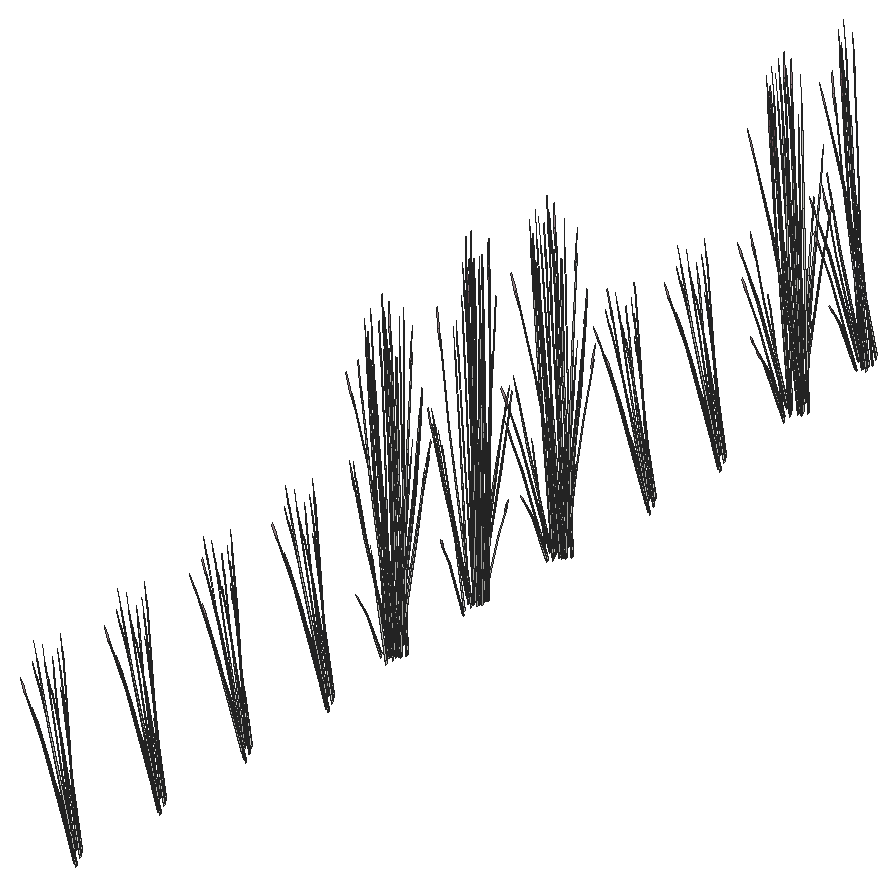
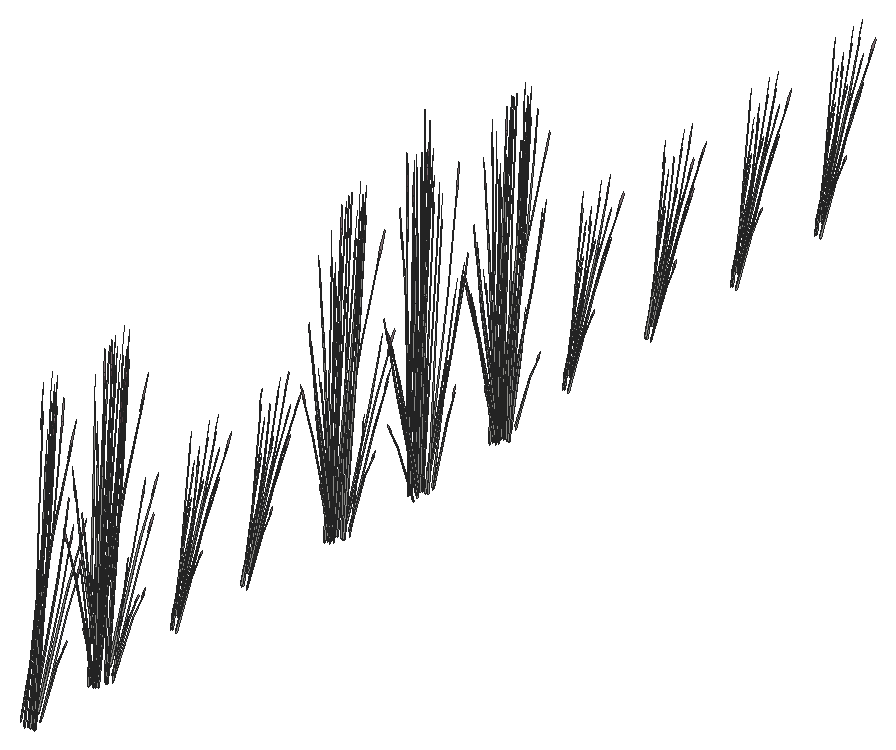
# SketchUp Ruby script. Lengths in inches.
U = 1.inch
M = Sketchup.active_model
def pt(a) = Geom::Point3d.new(a.map { |v| v * U })
def face(e, loops, mat)
  f = e.add_face(loops[0].map { |a| pt(a) })
  loops[1..].each { |l| e.add_face(l.map { |a| pt(a) }).erase! }
  f.material = f.back_material = mat if mat
  f
end
# faces: each face lists its corners as indices into pts; further lists are holes
def faces(e, pts, list, mat = nil) = list.each { |f| face(e, (f[0].is_a?(Array) ? f : [f]).map { |l| l.map { |i| pts[i] } }, mat) }
# xy, xz, yz: faces in a plane at the given z, y or x. An outline is a flat list of corners, or four numbers for a rectangle; further outlines are holes
def ring(l) = l.size == 4 ? [[l[0], l[1]], [l[2], l[1]], [l[2], l[3]], [l[0], l[3]]] : l.each_slice(2).to_a
def flat(e, list, mat, &to3) = list.each { |f| face(e, (f[0].is_a?(Array) ? f : [f]).map { |l| ring(l).map { |u, v| to3.(u, v) } }, mat) }
def xy(e, z, list, mat = nil) = flat(e, list, mat) { |x, y| [x, y, z] }
def xz(e, y, list, mat = nil) = flat(e, list, mat) { |x, z| [x, y, z] }
def yz(e, x, list, mat = nil) = flat(e, list, mat) { |y, z| [x, y, z] }
def lines(e, pts, list) = list.each { |a, b| e.add_line(pt(pts[a]), pt(pts[b])) }
# prism: a flat outline (further loops are holes) pulled along v
def prism(e, loops, v, mat = nil)
  f = face(e, loops, mat); d = Geom::Vector3d.new(v.map { |x| x * U })
  f.pushpull(f.normal.samedirection?(d) ? d.length : -d.length)
end
def box(e, o, s, mat = nil) = prism(e, [[o, [o[0] + s[0], o[1], o[2]], [o[0] + s[0], o[1] + s[1], o[2]], [o[0], o[1] + s[1], o[2]]]], [0, 0, s[2]], mat)
def at(x, y, z, deg = 0) = Geom::Transformation.translation(pt([x, y, z])) * Geom::Transformation.rotation(ORIGIN, Z_AXIS, deg.degrees)
def axes(o, x, y, z) = Geom::Transformation.new([*x, 0, *y, 0, *z, 0, *pt(o).to_a, 1])
def part(name) = M.definitions.add(name)
# library, detail: a bought-in or finely detailed component or shape, given as its bounding box
def library(name, o, s) = part(name).tap { |d| box(d.entities, o, s) }
def detail(e, o, s) = box(e.add_group.entities, o, s)
def put(e, d, t, mat = nil) = e.add_instance(d, t).tap { |i| i.material = mat if mat }
def group(e, t, mat = nil) = e.add_group.tap { |g| g.transformation = t; g.material = mat if mat }.entities
root = M.entities
M.materials.add("LightPink_Translucent").color = [144, 107, 117]
M.materials["LightPink_Translucent"].alpha = 0.75
c1 = part("blade")
p = [[2.15,0.21,22],[0,0.17,0],[0.09,0.45,0],[2.18,0.31,22],[2.29,0.31,22],[0.38,0.45,0],
  [2.48,0.24,33],[2.49,0.24,33],[2.48,0.22,33]]
faces(c1.entities,p,[[0,1,2,3],[4,5,2,3],[6,3,4,7],[8,0,3,6]])
c2 = part("seeds")
p = [[0.3,-0.1,1.38],[-0.01,-0.03,1.59],[-0.01,-0.03,0.03],[0.14,-0.07,-0.07],[0.29,-0.03,3],[0.15,0.01,3.11]]
faces(c2.entities,p,[[0,1,2,3],[1,0,4,5]],"LightPink_Translucent")
c3 = part("blade with seeds")
put(c3.entities,c1,at(0,0,0))
put(c3.entities,c2,axes([2.4,0.25,30.99],[1.5799,-0.05474,1.17369],[-0.12525,1.92788,0.29478],[-0.07173,-0.02425,1.56792]))
put(root,c3,axes([397.34,179.68,2.375],[-0.44133,0,0],[0,-0.52122,-0.51607],[0,-0.11871,1.63711]))
put(root,c3,axes([397.96,181,2.03],[-0.08291,-0.40636,-0.30978],[0.32928,-0.11539,0.30978],[-0.06638,-0.04686,1.38974]))
put(root,c3,axes([398.54,276.34,2.02],[-0.33032,-0.23318,-0.49651],[0.19744,-0.41812,0],[-0.07523,-0.05311,1.57504]))
put(root,c3,axes([398.4,272.86,1.49],[-0.03419,0.06144,1.76342],[-0.3455,0.13246,-0.26939],[-0.08346,-0.12049,0.30037]))
put(root,c3,axes([397.78,181.42,4.53],[-0.23881,0.24554,-0.35414],[-0.22606,-0.28036,0.4572],[-0.0344,0.14245,0.87481]))
put(root,c3,axes([398.2,290.38,2.59],[-0.02137,0.15256,1.43002],[-0.31245,0.12771,-0.30754],[-0.07303,-0.19719,0.61141]))
put(root,c3,axes([398.3,290.78,3.875],[0.08068,0.14973,1.71376],[-0.3728,0.12606,0.13857],[-0.08426,-0.23506,0.73262]))
put(root,c3,axes([398.74,276.62,2.375],[-0.22066,0.46731,0],[-0.36918,-0.26061,-0.51607],[-0.08408,-0.05936,1.63711]))
put(root,c3,axes([396.73,201.81,2.82],[0.32063,-0.08258,0.06507],[0.07371,0.33271,-0.86304],[-0.02033,0.16842,0.7736]))
put(root,c3,axes([398.24,200.32,2.67],[0.04113,0.53214,-0.29095],[-0.42835,0.03218,-0.50002],[-0.07543,0.07088,1.59708]))
put(root,c3,axes([397.28,199.42,2.1],[-0.14494,-0.47823,-0.69835],[0.41752,-0.17223,-0.18329],[-0.01602,-0.16194,1.54149]))
put(root,c3,axes([398.13,221,2.59],[0.11138,-0.07357,1.43002],[0.27499,0.22183,-0.30754],[-0.08185,0.19194,0.61141]))
put(root,c3,axes([400.46,100.5625,3.875],[0.14639,-0.01056,1.71376],[-0.09712,0.45778,0.13857],[-0.20862,-0.02831,0.73262]))
put(root,c3,axes([400.46,120.65,3.875],[0.14639,-0.01056,1.71376],[-0.09712,0.45778,0.13857],[-0.20862,-0.02831,0.73262]))
put(root,c3,axes([400.46,141.1,3.875],[0.14639,-0.01056,1.71376],[-0.09712,0.45778,0.13857],[-0.20862,-0.02831,0.73262]))
put(root,c3,axes([400.46,160.8,3.875],[0.14639,-0.01056,1.71376],[-0.09712,0.45778,0.13857],[-0.20862,-0.02831,0.73262]))
put(root,c3,axes([400.46,237.64,3.875],[0.14639,-0.01056,1.71376],[-0.09712,0.45778,0.13857],[-0.20862,-0.02831,0.73262]))
put(root,c3,axes([400.46,254.51,3.875],[0.14639,-0.01056,1.71376],[-0.09712,0.45778,0.13857],[-0.20862,-0.02831,0.73262]))
put(root,c3,axes([399,180.6875,2.06],[-0.23773,0.35053,-0.62353],[-0.29532,-0.31785,-0.16365],[-0.09526,0.08744,1.37633]))
put(root,c3,axes([397.93,197.92,4.68],[-0.34695,-0.11691,-0.51099],[0.11892,-0.40083,-0.3958],[-0.03181,-0.16138,0.97773]))
put(root,c3,axes([397.97,216.8,2.13],[-0.10181,0.3808,-0.03893],[-0.31336,-0.11714,-0.17649],[-0.04758,-0.06228,0.58215]))
put(root,c3,axes([398.44,290.7,4.53],[-0.05451,-0.37564,-0.35414],[0.31161,-0.09919,0.4572],[-0.0837,-0.10765,0.87481]))
put(root,c3,axes([397.57,292.6,2.375],[-0.44133,0,0],[0,-0.52122,-0.51607],[0,-0.11871,1.63711]))
put(root,c3,axes([397.68,179.54,2.33],[-0.32829,0.39208,0.30756],[-0.32849,-0.38796,-0.36492],[-0.01146,-0.11134,1.64885]))
put(root,c3,axes([397.29,200.9,3.875],[-0.00864,-0.17899,1.71376],[0.37441,0.11874,0.13857],[-0.02316,0.25508,0.73262]))
put(root,c3,axes([399.03,180.62,3.33],[0.305,0.18805,1.51261],[-0.29879,0.40513,0.59816],[-0.13384,-0.24012,1.26806]))
put(root,c3,axes([396.59,199.37,2.03],[0.24637,-0.29097,-0.30978],[0.24637,0.29097,0.30978],[0,-0.09372,1.38974]))
put(root,c3,axes([397.7,197.49,2.13],[-0.2439,0.26754,-0.03893],[-0.22348,-0.29302,-0.17649],[-0.01573,-0.08303,0.58215]))
put(root,c3,axes([398.4375,216.32,2.59],[-0.02137,0.15256,1.43002],[-0.31245,0.12771,-0.30754],[-0.07303,-0.19719,0.61141]))
put(root,c3,axes([397.87,177.21,2.77],[0.18411,0.16231,1.1486],[-0.26813,0.09757,0.84392],[-0.05737,-0.12474,0.25299]))
put(root,c3,axes([399.16,180.49,2.46],[-0.34464,-0.37536,-0.25192],[0.29,-0.42149,0.5513],[-0.0928,0.04391,1.68216]))
put(root,c3,axes([397.6,200.125,2.36],[0.44609,0.09826,0.45755],[-0.09078,0.55493,0.17955],[-0.06519,-0.05359,1.58856]))
put(root,c3,axes([398.54,216.72,3.875],[0.08068,0.14973,1.71376],[-0.3728,0.12606,0.13857],[-0.08426,-0.23506,0.73262]))
put(root,c3,axes([398.54,180.13,2.21],[-0.21202,-0.39143,-0.44739],[0.32115,-0.27564,0.21531],[-0.06861,-0.04843,1.43643]))
put(root,c3,axes([399.23,219.22,2.67],[-0.35635,0.30962,-0.29095],[-0.23697,-0.43749,-0.50002],[-0.08792,-0.04443,1.59708]))
put(root,c3,axes([398.34,277.29,2.59],[0.11138,-0.07357,1.43002],[0.27499,0.22183,-0.30754],[-0.08185,0.19194,0.61141]))
put(root,c3,axes([397.9375,181.16,5.34],[-0.00918,0.43138,-0.7886],[-0.38672,-0.02897,0.09517],[-0.04081,0.18275,1.11556]))
put(root,c3,axes([398.18,273.1,2.13],[-0.10181,0.3808,-0.03893],[-0.31336,-0.11714,-0.17649],[-0.04758,-0.06228,0.58215]))
put(root,c3,axes([398.67,216.64,4.53],[-0.05451,-0.37564,-0.35414],[0.31161,-0.09919,0.4572],[-0.0837,-0.10765,0.87481]))
put(root,c3,axes([397.93,182.38,2.77],[-0.00913,-0.2773,1.1486],[0.22824,0.19778,0.84392],[-0.04489,0.13217,0.25299]))
put(root,c3,axes([397.91,292.46,2.33],[-0.32829,0.39208,0.30756],[-0.32849,-0.38796,-0.36492],[-0.01146,-0.11134,1.64885]))
put(root,c3,axes([397.8,218.54,2.375],[-0.44133,0,0],[0,-0.52122,-0.51607],[0,-0.11871,1.63711]))
put(root,c3,axes([397.49,200.03,2.72],[-0.17124,0.42022,0.44739],[-0.35581,-0.20224,-0.21531],[0,-0.09687,1.43643]))
put(root,c3,axes([398.42,219.87,2.03],[-0.08291,-0.40636,-0.30978],[0.32928,-0.11539,0.30978],[-0.06638,-0.04686,1.38974]))
put(root,c3,axes([398.05,198,4.98],[-0.16845,-0.3792,-0.71045],[0.34676,-0.21133,0.08574],[-0.03939,-0.18322,1.00501]))
put(root,c3,axes([398.99,180.41,2.21],[-0.38326,0.02879,-0.44739],[-0.03466,-0.47788,0.21531],[-0.06861,0.04843,1.43643]))
put(root,c3,axes([399.26,293.55,3.33],[0.305,0.18805,1.51261],[-0.29879,0.40513,0.59816],[-0.13384,-0.24012,1.26806]))
put(root,c3,axes([398.24,220.29,4.53],[-0.23881,0.24554,-0.35414],[-0.22606,-0.28036,0.4572],[-0.0344,0.14245,0.87481]))
put(root,c3,axes([398.65,272.62,2.59],[-0.02137,0.15256,1.43002],[-0.31245,0.12771,-0.30754],[-0.07303,-0.19719,0.61141]))
put(root,c3,axes([400.52,101.37,3.875],[0.12246,-0.09864,1.71376],[0.1031,0.45582,0.13857],[-0.19225,0.10302,0.73262]))
put(root,c3,axes([400.52,121.46,3.875],[0.12246,-0.09864,1.71376],[0.1031,0.45582,0.13857],[-0.19225,0.10302,0.73262]))
put(root,c3,axes([400.52,141.91,3.875],[0.12246,-0.09864,1.71376],[0.1031,0.45582,0.13857],[-0.19225,0.10302,0.73262]))
put(root,c3,axes([400.52,161.6,3.875],[0.12246,-0.09864,1.71376],[0.1031,0.45582,0.13857],[-0.19225,0.10302,0.73262]))
put(root,c3,axes([400.52,238.44,3.875],[0.12246,-0.09864,1.71376],[0.1031,0.45582,0.13857],[-0.19225,0.10302,0.73262]))
put(root,c3,axes([400.52,255.32,3.875],[0.12246,-0.09864,1.71376],[0.1031,0.45582,0.13857],[-0.19225,0.10302,0.73262]))
put(root,c3,axes([398.75,273.01,3.875],[0.08068,0.14973,1.71376],[-0.3728,0.12606,0.13857],[-0.08426,-0.23506,0.73262]))
put(root,c3,axes([398.1,290.14,2.77],[0.18411,0.16231,1.1486],[-0.26813,0.09757,0.84392],[-0.05737,-0.12474,0.25299]))
put(root,c3,axes([399.4375,275.51,2.67],[-0.35635,0.30962,-0.29095],[-0.23697,-0.43749,-0.50002],[-0.08792,-0.04443,1.59708]))
put(root,c3,axes([400.14,102.14,2.59],[0.12266,0.03828,1.43002],[0.07906,0.39104,-0.30754],[-0.16661,0.0732,0.61141]))
put(root,c3,axes([400.14,122.24,2.59],[0.12266,0.03828,1.43002],[0.07906,0.39104,-0.30754],[-0.16661,0.0732,0.61141]))
put(root,c3,axes([400.14,142.68,2.59],[0.12266,0.03828,1.43002],[0.07906,0.39104,-0.30754],[-0.16661,0.0732,0.61141]))
put(root,c3,axes([400.14,162.38,2.59],[0.12266,0.03828,1.43002],[0.07906,0.39104,-0.30754],[-0.16661,0.0732,0.61141]))
put(root,c3,axes([400.14,239.22,2.59],[0.12266,0.03828,1.43002],[0.07906,0.39104,-0.30754],[-0.16661,0.0732,0.61141]))
put(root,c3,axes([400.14,256.1,2.59],[0.12266,0.03828,1.43002],[0.07906,0.39104,-0.30754],[-0.16661,0.0732,0.61141]))
put(root,c3,axes([397.37,201.01,2.47],[0.37926,-0.12378,0.17642],[0.09365,0.46065,0.35086],[-0.03382,-0.06712,1.60407]))
put(root,c3,axes([398.26,181.21,2.48],[0.33032,0.23318,0.49651],[-0.19744,0.41812,0],[-0.07523,-0.05311,1.57504]))
put(root,c3,axes([399.47,219.55,2.06],[-0.23773,0.35053,-0.62353],[-0.29532,-0.31785,-0.16365],[-0.09526,0.08744,1.37633]))
put(root,c3,axes([397.81,181.77,3.36],[0.00775,-0.24075,1.54345],[0.34877,0.12716,0.21329],[-0.03022,0.25658,0.72882]))
put(root,c3,axes([398.88,272.94,4.53],[-0.05451,-0.37564,-0.35414],[0.31161,-0.09919,0.4572],[-0.0837,-0.10765,0.87481]))
put(root,c3,axes([397.85,201.09,2.2],[-0.35581,-0.20937,0],[0.17124,-0.43505,0],[0,0,1.62707]))
put(root,c3,axes([398.01,274.84,2.375],[-0.44133,0,0],[0,-0.52122,-0.51607],[0,-0.11871,1.63711]))
put(root,c3,axes([398.63,276.16,2.03],[-0.08291,-0.40636,-0.30978],[0.32928,-0.11539,0.30978],[-0.06638,-0.04686,1.38974]))
put(root,c3,axes([398.57,180.36,2.4375],[0.09355,-0.55261,-0.23429],[0.44354,0.09633,0.51271],[-0.0775,-0.07631,1.5644]))
put(root,c3,axes([398.14,218.4,2.33],[-0.32829,0.39208,0.30756],[-0.32849,-0.38796,-0.36492],[-0.01146,-0.11134,1.64885]))
put(root,c3,axes([398.68,201.61,2.375],[0.22066,0.46731,0],[-0.36918,0.26061,-0.51607],[-0.08408,0.05936,1.63711]))
put(root,c3,axes([401.22,100.89,3.34],[0.10032,-0.06746,1.77064],[0.0346,0.47103,0.13857],[-0.2173,0.0625,0.63284]))
put(root,c3,axes([401.22,120.98,3.34],[0.10032,-0.06746,1.77064],[0.0346,0.47103,0.13857],[-0.2173,0.0625,0.63284]))
put(root,c3,axes([401.22,141.43,3.34],[0.10032,-0.06746,1.77064],[0.0346,0.47103,0.13857],[-0.2173,0.0625,0.63284]))
put(root,c3,axes([401.22,161.125,3.34],[0.10032,-0.06746,1.77064],[0.0346,0.47103,0.13857],[-0.2173,0.0625,0.63284]))
put(root,c3,axes([401.22,237.97,3.34],[0.10032,-0.06746,1.77064],[0.0346,0.47103,0.13857],[-0.2173,0.0625,0.63284]))
put(root,c3,axes([401.22,254.84,3.34],[0.10032,-0.06746,1.77064],[0.0346,0.47103,0.13857],[-0.2173,0.0625,0.63284]))
put(root,c3,axes([398.45,276.59,4.53],[-0.23881,0.24554,-0.35414],[-0.22606,-0.28036,0.4572],[-0.0344,0.14245,0.87481]))
put(root,c3,axes([399.5,219.49,3.33],[0.305,0.18805,1.51261],[-0.29879,0.40513,0.59816],[-0.13384,-0.24012,1.26806]))
put(root,c3,axes([398.73,180.49,2.62],[-0.06809,0.4162,0.1448],[-0.33266,-0.07225,-0.41347],[-0.06054,-0.04274,1.26744]))
put(root,c3,axes([398.33,216.08,2.77],[0.18411,0.16231,1.1486],[-0.26813,0.09757,0.84392],[-0.05737,-0.12474,0.25299]))
put(root,c3,axes([399.63,219.36,2.46],[-0.34464,-0.37536,-0.25192],[0.29,-0.42149,0.5513],[-0.0928,0.04391,1.68216]))
put(root,c3,axes([399.39,181.64,2.02],[-0.33032,0.23318,-0.49651],[-0.19744,-0.41812,0],[-0.07523,0.05311,1.57504]))
put(root,c3,axes([397.4375,179.32,2.02],[0,-0.46636,-0.49651],[0.39487,0,0],[0,-0.10622,1.57504]))
put(root,c3,axes([399,219,2.21],[-0.21202,-0.39143,-0.44739],[0.32115,-0.27564,0.21531],[-0.06861,-0.04843,1.43643]))
put(root,c3,axes([397.61,179.75,2.48],[0,0.46636,0.49651],[-0.39487,0,0],[0,-0.10622,1.57504]))
put(root,c3,axes([399.41,181.52,2.19],[-0.21791,-0.46895,-0.05142],[0.36918,-0.26061,0.51607],[-0.09097,0.04465,1.6363]))
put(root,c3,axes([399.68,275.85,2.06],[-0.23773,0.35053,-0.62353],[-0.29532,-0.31785,-0.16365],[-0.09526,0.08744,1.37633]))
put(root,c3,axes([398.49,201.04,2.47],[0.10196,-0.46348,0.17642],[0.3731,0.13116,0.35086],[-0.06445,0.00226,1.60407]))
put(root,c3,axes([398.32,200.42,2.62],[0.26075,0.2802,0.1448],[-0.2175,0.31612,-0.41347],[-0.06054,0.04274,1.26744]))
put(root,c3,axes([398.4,220.03,5.34],[-0.00918,0.43138,-0.7886],[-0.38672,-0.02897,0.09517],[-0.04081,0.18275,1.11556]))
put(root,c3,axes([398.35,274.7,2.33],[-0.32829,0.39208,0.30756],[-0.32849,-0.38796,-0.36492],[-0.01146,-0.11134,1.64885]))
put(root,c3,axes([398.23,200.08,2.3],[-0.32829,-0.4014,-0.06131],[0.32849,-0.40164,0],[-0.01146,-0.01402,1.75571]))
put(root,c3,axes([398.4,221.24,2.77],[-0.00913,-0.2773,1.1486],[0.22824,0.19778,0.84392],[-0.04489,0.13217,0.25299]))
put(root,c3,axes([398.8,293.28,2.4375],[0.09355,-0.55261,-0.23429],[0.44354,0.09633,0.51271],[-0.0775,-0.07631,1.5644]))
put(root,c3,axes([398.02,181.31,5],[0.25266,0.31335,-0.5672],[-0.2669,0.27442,-0.43934],[-0.03844,0.15921,1.08528]))
put(root,c3,axes([398.32,200.22,2.72],[0.38326,-0.02879,0.44739],[0.03466,0.47788,-0.21531],[-0.06861,0.04843,1.43643]))
put(root,c3,axes([399.45,219.28,2.21],[-0.38326,0.02879,-0.44739],[-0.03466,-0.47788,0.21531],[-0.06861,0.04843,1.43643]))
put(root,c3,axes([399.32,181.46,2.03],[-0.32928,-0.11539,-0.30978],[0.08291,-0.40636,0.30978],[-0.06638,0.04686,1.38974]))
put(root,c3,axes([399.71,275.78,3.33],[0.305,0.18805,1.51261],[-0.29879,0.40513,0.59816],[-0.13384,-0.24012,1.26806]))
put(root,c3,axes([400.89,100.14,4.98],[-0.35281,-0.01123,-0.71045],[0.0237,-0.47284,0.08574],[-0.14947,-0.0499,1.00501]))
put(root,c3,axes([400.89,120.23,4.98],[-0.35281,-0.01123,-0.71045],[0.0237,-0.47284,0.08574],[-0.14947,-0.0499,1.00501]))
put(root,c3,axes([400.89,140.68,4.98],[-0.35281,-0.01123,-0.71045],[0.0237,-0.47284,0.08574],[-0.14947,-0.0499,1.00501]))
put(root,c3,axes([400.89,160.37,4.98],[-0.35281,-0.01123,-0.71045],[0.0237,-0.47284,0.08574],[-0.14947,-0.0499,1.00501]))
put(root,c3,axes([400.89,237.21,4.98],[-0.35281,-0.01123,-0.71045],[0.0237,-0.47284,0.08574],[-0.14947,-0.0499,1.00501]))
put(root,c3,axes([400.89,254.09,4.98],[-0.35281,-0.01123,-0.71045],[0.0237,-0.47284,0.08574],[-0.14947,-0.0499,1.00501]))
put(root,c3,axes([398.41,201.32,2.33],[0.44186,0.15158,0.30756],[-0.11054,0.54181,-0.36492],[-0.07313,0.06781,1.64885]))
put(root,c3,axes([398.47,179.86,2.67],[-0.39748,-0.22252,-0.29095],[0.19139,-0.46966,-0.50002],[-0.01249,-0.11531,1.59708]))
put(root,c3,axes([397.76,197.16,1.49],[-0.0592,0.0168,1.76342],[-0.32738,-0.18913,-0.26939],[0.00549,-0.15776,0.30037]))
put(root,c3,axes([399.5,179.72,2.84],[-0.00964,-0.43909,1.41272],[0.43635,0.11382,0.59816],[-0.1032,0.24027,1.3335]))
put(root,c3,axes([398.54,272.375,2.77],[0.18411,0.16231,1.1486],[-0.26813,0.09757,0.84392],[-0.05737,-0.12474,0.25299]))
put(root,c3,axes([399.84,275.65,2.46],[-0.34464,-0.37536,-0.25192],[0.29,-0.42149,0.5513],[-0.0928,0.04391,1.68216]))
put(root,c3,axes([400.61,100.25,2.59],[0.06891,0.12984,1.43002],[-0.15879,0.35293,-0.30754],[-0.16304,-0.08436,0.61141]))
put(root,c3,axes([400.61,120.34,2.59],[0.06891,0.12984,1.43002],[-0.15879,0.35293,-0.30754],[-0.16304,-0.08436,0.61141]))
put(root,c3,axes([400.61,140.79,2.59],[0.06891,0.12984,1.43002],[-0.15879,0.35293,-0.30754],[-0.16304,-0.08436,0.61141]))
put(root,c3,axes([400.61,160.49,2.59],[0.06891,0.12984,1.43002],[-0.15879,0.35293,-0.30754],[-0.16304,-0.08436,0.61141]))
put(root,c3,axes([400.61,237.33,2.59],[0.06891,0.12984,1.43002],[-0.15879,0.35293,-0.30754],[-0.16304,-0.08436,0.61141]))
put(root,c3,axes([400.61,254.2,2.59],[0.06891,0.12984,1.43002],[-0.15879,0.35293,-0.30754],[-0.16304,-0.08436,0.61141]))
put(root,c3,axes([399.21,275.29,2.21],[-0.21202,-0.39143,-0.44739],[0.32115,-0.27564,0.21531],[-0.06861,-0.04843,1.43643]))
put(root,c3,axes([397.66,292.25,2.02],[0,-0.46636,-0.49651],[0.39487,0,0],[0,-0.10622,1.57504]))
put(root,c3,axes([397.83,292.68,2.48],[0,0.46636,0.49651],[-0.39487,0,0],[0,-0.10622,1.57504]))
put(root,c3,axes([398.6,201.29,2.48],[0.33032,-0.23318,0.49651],[0.19744,0.41812,0],[-0.07523,0.05311,1.57504]))
put(root,c3,axes([398.61,276.33,5.34],[-0.00918,0.43138,-0.7886],[-0.38672,-0.02897,0.09517],[-0.04081,0.18275,1.11556]))
put(root,c3,axes([400.33,100.95,4.53],[-0.29332,-0.1301,-0.35414],[0.08555,-0.37955,0.4572],[-0.11809,0.0348,0.87481]))
put(root,c3,axes([400.33,121.05,4.53],[-0.29332,-0.1301,-0.35414],[0.08555,-0.37955,0.4572],[-0.11809,0.0348,0.87481]))
put(root,c3,axes([400.33,141.49,4.53],[-0.29332,-0.1301,-0.35414],[0.08555,-0.37955,0.4572],[-0.11809,0.0348,0.87481]))
put(root,c3,axes([400.33,161.1875,4.53],[-0.29332,-0.1301,-0.35414],[0.08555,-0.37955,0.4572],[-0.11809,0.0348,0.87481]))
put(root,c3,axes([400.33,238.03,4.53],[-0.29332,-0.1301,-0.35414],[0.08555,-0.37955,0.4572],[-0.11809,0.0348,0.87481]))
put(root,c3,axes([400.33,254.91,4.53],[-0.29332,-0.1301,-0.35414],[0.08555,-0.37955,0.4572],[-0.11809,0.0348,0.87481]))
put(root,c3,axes([398.09,197.68,4.53],[0.1064,-0.35863,-0.35414],[0.31043,0.1046,0.4572],[-0.02846,-0.14439,0.87481]))
put(root,c3,axes([397.57,199.61,2.36],[0.15345,0.52148,0.45755],[-0.43845,0.18134,0.17955],[0.00536,-0.09582,1.58856]))
put(root,c3,axes([398.72,220.08,2.48],[0.33032,0.23318,0.49651],[-0.19744,0.41812,0],[-0.07523,-0.05311,1.57504]))
put(root,c3,axes([400.73,99.83,3.875],[0.1311,0.08035,1.71376],[-0.27131,0.33708,0.13857],[-0.16909,-0.15206,0.73262]))
put(root,c3,axes([400.73,119.92,3.875],[0.1311,0.08035,1.71376],[-0.27131,0.33708,0.13857],[-0.16909,-0.15206,0.73262]))
put(root,c3,axes([400.73,140.37,3.875],[0.1311,0.08035,1.71376],[-0.27131,0.33708,0.13857],[-0.16909,-0.15206,0.73262]))
put(root,c3,axes([400.73,160.0625,3.875],[0.1311,0.08035,1.71376],[-0.27131,0.33708,0.13857],[-0.16909,-0.15206,0.73262]))
put(root,c3,axes([400.73,236.9,3.875],[0.1311,0.08035,1.71376],[-0.27131,0.33708,0.13857],[-0.16909,-0.15206,0.73262]))
put(root,c3,axes([400.73,253.78,3.875],[0.1311,0.08035,1.71376],[-0.27131,0.33708,0.13857],[-0.16909,-0.15206,0.73262]))
put(root,c3,axes([398.27,220.64,3.36],[0.00775,-0.24075,1.54345],[0.34877,0.12716,0.21329],[-0.03022,0.25658,0.72882]))
put(root,c3,axes([397.5,199.55,2.21],[0.17124,-0.42022,-0.44739],[0.35581,0.20224,0.21531],[0,-0.09687,1.43643]))
put(root,c3,axes([398.61,277.54,2.77],[-0.00913,-0.2773,1.1486],[0.22824,0.19778,0.84392],[-0.04489,0.13217,0.25299]))
put(root,c3,axes([397.93,200.9,2.2],[-0.11516,-0.40207,0],[0.32884,-0.1408,0],[0,0,1.54371]))
put(root,c3,axes([397.52,201.75,1.49],[0.05712,-0.02538,1.76342],[0.34359,0.13968,-0.26939],[0.01005,0.15742,0.30037]))
put(root,c3,axes([397.74,181.78,2.82],[0.32063,-0.08258,0.06507],[0.07371,0.33271,-0.86304],[-0.02033,0.16842,0.7736]))
put(root,c3,axes([399.03,219.22,2.4375],[0.09355,-0.55261,-0.23429],[0.44354,0.09633,0.51271],[-0.0775,-0.07631,1.5644]))
put(root,c3,axes([399.66,275.57,2.21],[-0.38326,0.02879,-0.44739],[-0.03466,-0.47788,0.21531],[-0.06861,0.04843,1.43643]))
put(root,c3,axes([399.26,180.28,2.67],[0.04113,0.53214,-0.29095],[-0.42835,0.03218,-0.50002],[-0.07543,0.07088,1.59708]))
put(root,c3,axes([398.29,179.39,2.1],[-0.14494,-0.47823,-0.69835],[0.41752,-0.17223,-0.18329],[-0.01602,-0.16194,1.54149]))
put(root,c3,axes([397.59,201.89,4.53],[-0.1064,0.35863,-0.35414],[-0.31043,-0.1046,0.4572],[0.02846,0.14439,0.87481]))
put(root,c3,axes([398.94,177.89,4.68],[-0.34695,-0.11691,-0.51099],[0.11892,-0.40083,-0.3958],[-0.03181,-0.16138,0.97773]))
put(root,c3,axes([399.2,219.35,2.62],[-0.06809,0.4162,0.1448],[-0.33266,-0.07225,-0.41347],[-0.06054,-0.04274,1.26744]))
put(root,c3,axes([400.53,101.15,4.68],[-0.09562,0.42421,-0.51099],[-0.32782,-0.1454,-0.3958],[-0.13199,0.0389,0.97773]))
put(root,c3,axes([400.53,121.24,4.68],[-0.09562,0.42421,-0.51099],[-0.32782,-0.1454,-0.3958],[-0.13199,0.0389,0.97773]))
put(root,c3,axes([400.53,141.6875,4.68],[-0.09562,0.42421,-0.51099],[-0.32782,-0.1454,-0.3958],[-0.13199,0.0389,0.97773]))
put(root,c3,axes([400.53,161.38,4.68],[-0.09562,0.42421,-0.51099],[-0.32782,-0.1454,-0.3958],[-0.13199,0.0389,0.97773]))
put(root,c3,axes([400.53,238.22,4.68],[-0.09562,0.42421,-0.51099],[-0.32782,-0.1454,-0.3958],[-0.13199,0.0389,0.97773]))
put(root,c3,axes([400.53,255.1,4.68],[-0.09562,0.42421,-0.51099],[-0.32782,-0.1454,-0.3958],[-0.13199,0.0389,0.97773]))
put(root,c3,axes([398.7,292.79,2.67],[-0.39748,-0.22252,-0.29095],[0.19139,-0.46966,-0.50002],[-0.01249,-0.11531,1.59708]))
put(root,c3,axes([398.3,180.86,3.875],[-0.00864,-0.17899,1.71376],[0.37441,0.11874,0.13857],[-0.02316,0.25508,0.73262]))
put(root,c3,axes([399.86,220.51,2.02],[-0.33032,0.23318,-0.49651],[-0.19744,-0.41812,0],[-0.07523,0.05311,1.57504]))
put(root,c3,axes([397.9,218.1875,2.02],[0,-0.46636,-0.49651],[0.39487,0,0],[0,-0.10622,1.57504]))
put(root,c3,axes([398.07,218.62,2.48],[0,0.46636,0.49651],[-0.39487,0,0],[0,-0.10622,1.57504]))
put(root,c3,axes([399.88,220.39,2.19],[-0.21791,-0.46895,-0.05142],[0.36918,-0.26061,0.51607],[-0.09097,0.04465,1.6363]))
put(root,c3,axes([400.78,100.23,4.68],[-0.25628,0.30892,-0.51099],[-0.22444,-0.32634,-0.3958],[-0.13021,-0.047,0.97773]))
put(root,c3,axes([400.78,120.32,4.68],[-0.25628,0.30892,-0.51099],[-0.22444,-0.32634,-0.3958],[-0.13021,-0.047,0.97773]))
put(root,c3,axes([400.78,140.77,4.68],[-0.25628,0.30892,-0.51099],[-0.22444,-0.32634,-0.3958],[-0.13021,-0.047,0.97773]))
put(root,c3,axes([400.78,160.47,4.68],[-0.25628,0.30892,-0.51099],[-0.22444,-0.32634,-0.3958],[-0.13021,-0.047,0.97773]))
put(root,c3,axes([400.78,237.31,4.68],[-0.25628,0.30892,-0.51099],[-0.22444,-0.32634,-0.3958],[-0.13021,-0.047,0.97773]))
put(root,c3,axes([400.78,254.19,4.68],[-0.25628,0.30892,-0.51099],[-0.22444,-0.32634,-0.3958],[-0.13021,-0.047,0.97773]))
put(root,c3,axes([398.93,276.375,2.48],[0.33032,0.23318,0.49651],[-0.19744,0.41812,0],[-0.07523,-0.05311,1.57504]))
put(root,c3,axes([397.61,179.33,2.03],[0.24637,-0.29097,-0.30978],[0.24637,0.29097,0.30978],[0,-0.09372,1.38974]))
put(root,c3,axes([400.36,101.12,1.49],[0.00895,0.0735,1.76342],[-0.18044,0.38382,-0.26939],[-0.12817,-0.01935,0.30037]))
put(root,c3,axes([400.36,121.21,1.49],[0.00895,0.0735,1.76342],[-0.18044,0.38382,-0.26939],[-0.12817,-0.01935,0.30037]))
put(root,c3,axes([400.36,141.66,1.49],[0.00895,0.0735,1.76342],[-0.18044,0.38382,-0.26939],[-0.12817,-0.01935,0.30037]))
put(root,c3,axes([400.36,161.36,1.49],[0.00895,0.0735,1.76342],[-0.18044,0.38382,-0.26939],[-0.12817,-0.01935,0.30037]))
put(root,c3,axes([400.36,238.2,1.49],[0.00895,0.0735,1.76342],[-0.18044,0.38382,-0.26939],[-0.12817,-0.01935,0.30037]))
put(root,c3,axes([400.36,255.08,1.49],[0.00895,0.0735,1.76342],[-0.18044,0.38382,-0.26939],[-0.12817,-0.01935,0.30037]))
put(root,c3,axes([398.48,276.93,3.36],[0.00775,-0.24075,1.54345],[0.34877,0.12716,0.21329],[-0.03022,0.25658,0.72882]))
put(root,c3,axes([398.72,177.45,2.13],[-0.2439,0.26754,-0.03893],[-0.22348,-0.29302,-0.17649],[-0.01573,-0.08303,0.58215]))
put(root,c3,axes([398.62,180.09,2.36],[0.44609,0.09826,0.45755],[-0.09078,0.55493,0.17955],[-0.06519,-0.05359,1.58856]))
put(root,c3,axes([399.24,275.52,2.4375],[0.09355,-0.55261,-0.23429],[0.44354,0.09633,0.51271],[-0.0775,-0.07631,1.5644]))
put(root,c3,axes([398.4,200.11,2.21],[-0.17124,0.42022,-0.44739],[-0.35581,-0.20224,0.21531],[0,0.09687,1.43643]))
put(root,c3,axes([398.48,220.17,5],[0.25266,0.31335,-0.5672],[-0.2669,0.27442,-0.43934],[-0.03844,0.15921,1.08528]))
put(root,c3,axes([398.52,292.31,2.1],[-0.14494,-0.47823,-0.69835],[0.41752,-0.17223,-0.18329],[-0.01602,-0.16194,1.54149]))
put(root,c3,axes([399.17,290.8125,4.68],[-0.34695,-0.11691,-0.51099],[0.11892,-0.40083,-0.3958],[-0.03181,-0.16138,0.97773]))
put(root,c3,axes([399.78,220.33,2.03],[-0.32928,-0.11539,-0.30978],[0.08291,-0.40636,0.30978],[-0.06638,0.04686,1.38974]))
put(root,c3,axes([399.4,275.65,2.62],[-0.06809,0.4162,0.1448],[-0.33266,-0.07225,-0.41347],[-0.06054,-0.04274,1.26744]))
put(root,c3,axes([398.93,218.73,2.67],[-0.39748,-0.22252,-0.29095],[0.19139,-0.46966,-0.50002],[-0.01249,-0.11531,1.59708]))
put(root,c3,axes([399.97,218.59,2.84],[-0.00964,-0.43909,1.41272],[0.43635,0.11382,0.59816],[-0.1032,0.24027,1.3335]))
put(root,c3,axes([399.08,199.85,2.47],[-0.2773,-0.3397,0.17642],[0.27945,-0.32949,0.35086],[-0.03063,0.06937,1.60407]))
put(root,c3,axes([399.88,102.96,2.77],[0.14709,-0.21136,1.1486],[0.05804,0.3346,0.84392],[-0.1063,0.05991,0.25299]))
put(root,c3,axes([399.88,123.05,2.77],[0.14709,-0.21136,1.1486],[0.05804,0.3346,0.84392],[-0.1063,0.05991,0.25299]))
put(root,c3,axes([399.88,143.5,2.77],[0.14709,-0.21136,1.1486],[0.05804,0.3346,0.84392],[-0.1063,0.05991,0.25299]))
put(root,c3,axes([399.88,163.2,2.77],[0.14709,-0.21136,1.1486],[0.05804,0.3346,0.84392],[-0.1063,0.05991,0.25299]))
put(root,c3,axes([399.88,240.04,2.77],[0.14709,-0.21136,1.1486],[0.05804,0.3346,0.84392],[-0.1063,0.05991,0.25299]))
put(root,c3,axes([399.88,256.92,2.77],[0.14709,-0.21136,1.1486],[0.05804,0.3346,0.84392],[-0.1063,0.05991,0.25299]))
put(root,c3,axes([398.51,179.99,2.72],[-0.17124,0.42022,0.44739],[-0.35581,-0.20224,-0.21531],[0,-0.09687,1.43643]))
put(root,c3,axes([399.07,177.96,4.98],[-0.16845,-0.3792,-0.71045],[0.34676,-0.21133,0.08574],[-0.03939,-0.18322,1.00501]))
put(root,c3,axes([400.07,276.81,2.02],[-0.33032,0.23318,-0.49651],[-0.19744,-0.41812,0],[-0.07523,0.05311,1.57504]))
put(root,c3,axes([398.11,274.48,2.02],[0,-0.46636,-0.49651],[0.39487,0,0],[0,-0.10622,1.57504]))
put(root,c3,axes([398.28,274.92,2.48],[0,0.46636,0.49651],[-0.39487,0,0],[0,-0.10622,1.57504]))
put(root,c3,axes([400.09,276.68,2.19],[-0.21791,-0.46895,-0.05142],[0.36918,-0.26061,0.51607],[-0.09097,0.04465,1.6363]))
put(root,c3,axes([398.12,199.66,2.21],[0,-0.53961,0],[0.44133,0,0],[0,0,1.79456]))
put(root,c3,axes([397.83,292.26,2.03],[0.24637,-0.29097,-0.30978],[0.24637,0.29097,0.30978],[0,-0.09372,1.38974]))
put(root,c3,axes([397.71,199.76,2.43],[0.39767,0.22603,0.24065],[-0.19139,0.46966,0.50002],[0,-0.10827,1.60543]))
